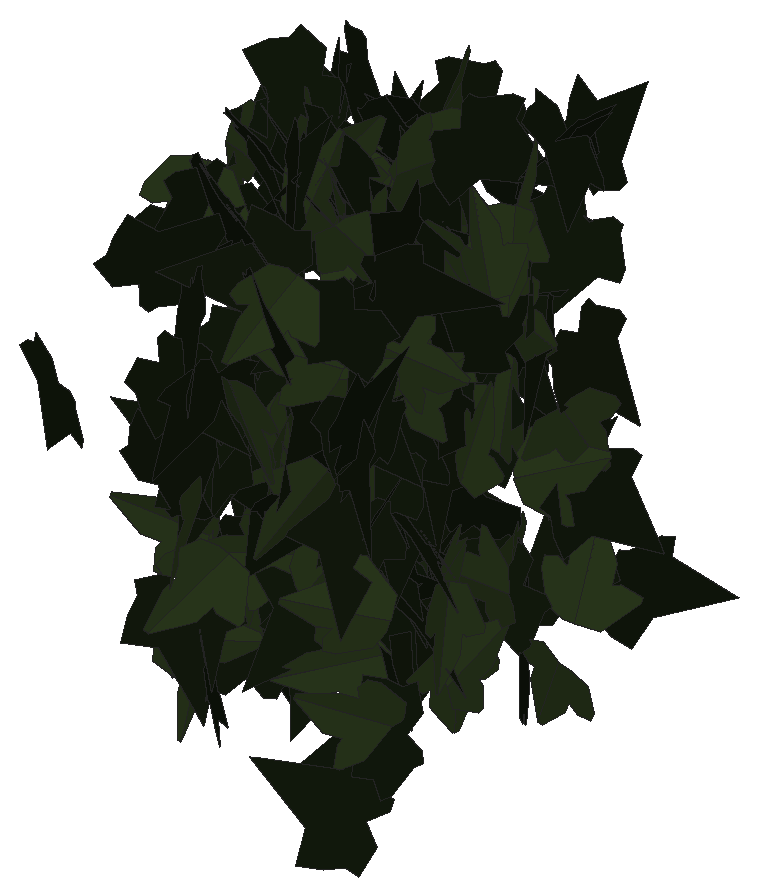
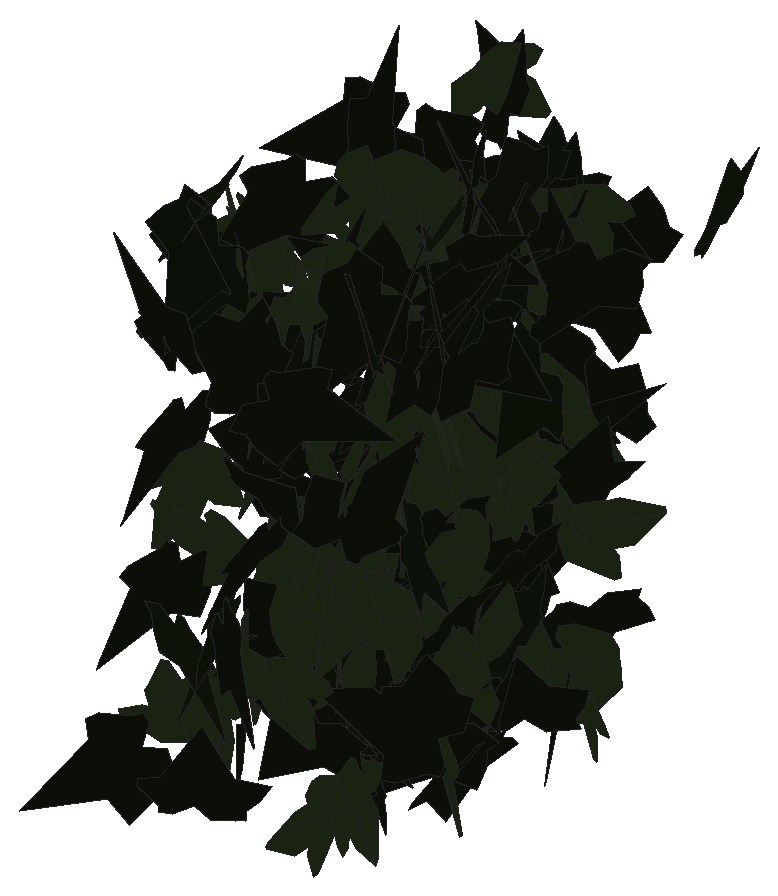
# SketchUp Ruby script. Lengths in inches.
U = 1.inch
M = Sketchup.active_model
def pt(a) = Geom::Point3d.new(a.map { |v| v * U })
def face(e, loops, mat)
  f = e.add_face(loops[0].map { |a| pt(a) })
  loops[1..].each { |l| e.add_face(l.map { |a| pt(a) }).erase! }
  f.material = f.back_material = mat if mat
  f
end
# faces: each face lists its corners as indices into pts; further lists are holes
def faces(e, pts, list, mat = nil) = list.each { |f| face(e, (f[0].is_a?(Array) ? f : [f]).map { |l| l.map { |i| pts[i] } }, mat) }
# xy, xz, yz: faces in a plane at the given z, y or x. An outline is a flat list of corners, or four numbers for a rectangle; further outlines are holes
def ring(l) = l.size == 4 ? [[l[0], l[1]], [l[2], l[1]], [l[2], l[3]], [l[0], l[3]]] : l.each_slice(2).to_a
def flat(e, list, mat, &to3) = list.each { |f| face(e, (f[0].is_a?(Array) ? f : [f]).map { |l| ring(l).map { |u, v| to3.(u, v) } }, mat) }
def xy(e, z, list, mat = nil) = flat(e, list, mat) { |x, y| [x, y, z] }
def xz(e, y, list, mat = nil) = flat(e, list, mat) { |x, z| [x, y, z] }
def yz(e, x, list, mat = nil) = flat(e, list, mat) { |y, z| [x, y, z] }
def lines(e, pts, list) = list.each { |a, b| e.add_line(pt(pts[a]), pt(pts[b])) }
# prism: a flat outline (further loops are holes) pulled along v
def prism(e, loops, v, mat = nil)
  f = face(e, loops, mat); d = Geom::Vector3d.new(v.map { |x| x * U })
  f.pushpull(f.normal.samedirection?(d) ? d.length : -d.length)
end
def box(e, o, s, mat = nil) = prism(e, [[o, [o[0] + s[0], o[1], o[2]], [o[0] + s[0], o[1] + s[1], o[2]], [o[0], o[1] + s[1], o[2]]]], [0, 0, s[2]], mat)
def at(x, y, z, deg = 0) = Geom::Transformation.translation(pt([x, y, z])) * Geom::Transformation.rotation(ORIGIN, Z_AXIS, deg.degrees)
def axes(o, x, y, z) = Geom::Transformation.new([*x, 0, *y, 0, *z, 0, *pt(o).to_a, 1])
def part(name) = M.definitions.add(name)
# library, detail: a bought-in or finely detailed component or shape, given as its bounding box
def library(name, o, s) = part(name).tap { |d| box(d.entities, o, s) }
def detail(e, o, s) = box(e.add_group.entities, o, s)
def put(e, d, t, mat = nil) = e.add_instance(d, t).tap { |i| i.material = mat if mat }
def group(e, t, mat = nil) = e.add_group.tap { |g| g.transformation = t; g.material = mat if mat }.entities
root = M.entities
M.materials.add("efeu1").color = [18, 25, 13]
M.materials.add("efeu2").color = [43, 57, 29]
c1 = part("ivyleaf_9")
p = [[1.54,2.16,1.25],[1.36,2.04,1.19],[-0.21,0.99,0.68],[-0.71,1.11,0.82],[-0.85,0.86,0.67],[-0.8,0.17,0.21],
  [-0.9,-0.01,0.1],[-0.67,-0.16,-0.02],[-0.08,-0.08,-0.05],[-0.03,-0.6,-0.4],[0.65,-0.88,-0.66],[0.83,-0.6,-0.49],
  [1.29,-0.42,-0.43],[1.8125,-0.07,-0.26],[1.21,0.44,0.15]]
faces(c1.entities,p,[[0,1,2,3,4,5,6,7,8,9,10,11,12,13,14]],"efeu1")
c2 = part("ivyleaf_10")
p = [[0,0.5,-0.03],[-0.0625,2.02,-0.43],[-0.19,2.01,-0.46],[-0.54,1.05,-0.29],[-0.52,0.625,-0.18],[-0.83,0.76,-0.28],
  [-1.16,0.64,-0.33],[-1.15,0.33,-0.24],[-0.77,-0.39,0.02],[-0.3,-0.51,0.16],[0.04,-0.48,0.23],[-0.02,2.01,-0.4375],
  [-0.06,2.01,-0.43],[0.04,-0.49,0.23],[0.67,-0.49,0.14],[1.38,0.36,-0.2],[1.375,0.51,-0.24],[0.81,0.65,-0.19],
  [0.62,0.59,-0.15],[0.6,1.09,-0.28],[0.5,1.23,-0.31]]
faces(c2.entities,p,[[0,1,2,3,4,5,6,7,8,9,10],[11,12,0,13,14,15,16,17,18,19,20]],"efeu2")
put(root,c1,axes([31.6875,223.98,213.96],[-0.33747,-0.32736,0.17014],[-0.11694,-0.12378,-0.47011],[0.34991,-0.35709,0.00698]))
put(root,c1,axes([31.4375,221.77,213.03],[-0.01587,-0.27679,-0.41609],[0.04585,0.41374,-0.27698],[0.49764,-0.04695,0.01225]))
put(root,c2,axes([31.33,222.96,213.41],[0.06539,-0.12843,-0.47878],[0.30609,-0.3694,0.14089],[-0.38991,-0.31152,0.03031]))
put(root,c1,axes([31.81,221.8,210.03],[-0.3415,-0.32972,0.15703],[0.11823,0.1036,0.47465],[-0.34554,0.36132,0.00721]))
put(root,c2,axes([31.98,221.37,209.31],[-0.14783,-0.03082,-0.47665],[-0.46593,-0.10055,0.151],[-0.10516,0.48881,0.00101]))
put(root,c2,axes([31.57,224.38,211.75],[0.2481,-0.43409,-0.00389],[0.0025,-0.00306,0.49998],[-0.4341,-0.24811,0.00065]))
put(root,c2,axes([31.63,222.88,210.6],[-0.00162,0.11657,-0.48622],[-0.04741,-0.48407,-0.11589],[-0.49774,0.04573,0.01262]))
put(root,c1,axes([31.56,224.39,209.48],[-0.06194,-0.46788,0.16508],[-0.02755,-0.16286,-0.47193],[0.49538,-0.06756,-0.0056]))
put(root,c1,axes([31.375,224.01,212.62],[0.48534,0.05286,-0.10793],[0.10585,0.02454,0.48805],[0.0569,-0.49659,0.01263]))
put(root,c1,axes([31.6875,224.75,210.8],[-0.29345,0.16275,-0.37067],[0.3272,-0.17423,-0.33554],[-0.23838,-0.43949,-0.00425]))
put(root,c2,axes([31.4,224.05,208.94],[0.3357,-0.12424,-0.3491],[0.3321,-0.10805,0.35782],[-0.16435,-0.47211,0.00998]))
put(root,c1,axes([31.87,223.68,212.84],[-0.0005,0.11983,-0.48543],[-0.0203,-0.48503,-0.11972],[-0.49959,0.01959,0.00535]))
put(root,c1,axes([31.8125,222.31,211.74],[0.04684,0.37913,0.3226],[0.03612,0.32058,-0.382],[-0.49649,0.05909,0.00264]))
put(root,c1,axes([31.875,225.68,211.17],[0.10776,0.10707,0.47636],[-0.43164,-0.2071,0.1442],[0.22819,-0.44232,0.0478]))
put(root,c1,axes([31.89,224.11,213.38],[-0.02238,-0.40573,-0.29134],[-0.01936,-0.29071,0.40634],[-0.49912,0.02947,-0.0027]))
put(root,c1,axes([31.54,224.39,213.21],[-0.03654,0.22317,0.44594],[0.07138,-0.44019,0.22614],[0.49353,0.08019,0.00031]))
put(root,c2,axes([31.41,225.27,210.07],[-0.21676,0.08364,-0.44274],[0.41102,-0.16459,-0.23232],[-0.1846,-0.46467,0.0026]))
put(root,c1,axes([31.57,222.9,209.77],[0.16919,-0.41329,-0.22487],[-0.08353,0.20879,-0.44658],[0.46303,0.18868,0.0016]))
put(root,c1,axes([31.86,224.08,212.77],[0.00119,-0.49676,0.05684],[0.03122,0.0568,0.49578],[-0.49902,0.00237,0.03115]))
put(root,c2,axes([31.78,223.5625,210.01],[0.05454,-0.15211,0.47317],[-0.11922,0.45811,0.16101],[-0.48251,-0.13038,0.0137]))
put(root,c2,axes([31.79,221.69,213.65],[0.44104,0.2007,-0.1233],[-0.11246,-0.05056,-0.48456],[-0.20697,0.45515,0.00054]))
put(root,c2,axes([31.75,222.37,210.68],[0.03924,0.41759,0.27217],[0.01727,0.27171,-0.41937],[-0.49816,0.04231,0.0069]))
put(root,c2,axes([31.79,221.63,207.48],[0.4189,-0.26458,0.06722],[0.05738,-0.03504,-0.49546],[0.26689,0.42281,0.00101]))
put(root,c1,axes([31.6,220.93,212.64],[-0.04412,-0.02615,0.49736],[0.48102,0.1272,0.04936],[-0.12911,0.48284,0.01393]))
put(root,c1,axes([31.58,223,208.71],[0.06296,-0.27116,0.41534],[0.15597,-0.38662,-0.27605],[0.47086,0.16432,0.0359]))
put(root,c1,axes([31.99,221.86,213.51],[-0.02515,0.05008,-0.49685],[0.05384,-0.49431,-0.05255],[-0.49646,-0.05614,0.01947]))
put(root,c2,axes([32.01,223.83,207.62],[0.30138,-0.30171,-0.26104],[-0.17078,0.19809,-0.42614],[0.36056,0.34602,0.01635]))
put(root,c1,axes([31.86,224.37,214.11],[0.30513,-0.19859,-0.34272],[-0.29281,0.17825,-0.36399],[0.26675,0.42283,-0.00752]))
put(root,c2,axes([31.85,225.26,211.94],[-0.14818,0.46373,-0.11399],[0.03283,-0.10917,-0.48683],[-0.47641,-0.15176,0.0019]))
put(root,c1,axes([31.58,223.63,213.24],[0.27836,-0.32305,0.26106],[0.18025,-0.18917,-0.42629],[0.37419,0.33144,0.01115]))
put(root,c1,axes([31.53,224.53,208.22],[0.21128,-0.08624,0.44489],[0.44522,-0.05202,-0.22152],[0.08449,0.48975,0.05481]))
put(root,c2,axes([31.98,224.79,212.15],[-0.03583,-0.15054,-0.47545],[-0.12988,-0.45741,0.15462],[-0.48151,0.13458,-0.00633]))
put(root,c2,axes([32,225.25,212.0625],[-0.2445,0.39048,0.19429],[-0.10854,0.16125,-0.46067],[-0.42242,-0.26744,0.00592]))
put(root,c1,axes([31.8125,221.43,208.35],[-0.10098,-0.44105,-0.21278],[0.05253,0.20625,-0.45244],[0.48687,-0.11373,0.00468]))
put(root,c1,axes([31.79,223.7,207.39],[0.03275,-0.49311,-0.07595],[-0.00644,0.07569,-0.4942],[0.49888,0.03335,-0.00139]))
put(root,c2,axes([31.93,225.46,210.32],[-0.1341,-0.40709,-0.25748],[0.10901,0.23469,-0.42783],[0.46918,-0.17088,0.02581]))
put(root,c2,axes([31.65,221.5,207.76],[-0.04159,-0.0317,-0.49726],[0.44458,0.22294,-0.0514],[0.22498,-0.44642,0.00965]))
put(root,c2,axes([32.05,226.7,209.76],[0.46811,0.08876,-0.15165],[-0.14956,-0.02529,-0.47644],[-0.09225,0.49141,0.00288]))
put(root,c2,axes([31.8125,221.9,210.1],[0.36867,-0.20175,0.27089],[0.23709,-0.13104,-0.42026],[0.24057,0.43832,-0.00096]))
put(root,c2,axes([31.63,221.86,211.14],[0.16871,0.04916,0.4681],[0.45456,0.11199,-0.17559],[-0.12211,0.48481,-0.0069]))
put(root,c1,axes([31.875,224.4,212.93],[0.49003,0.0694,-0.07107],[-0.07051,-0.00894,-0.49492],[-0.06996,0.49508,0.00102]))
put(root,c2,axes([31.96,223.61,213.27],[-0.20873,0.26397,0.36979],[0.21214,-0.30325,0.33621],[0.40178,0.29725,0.0146]))
put(root,c1,axes([32.36,221.36,210.33],[-0.22809,-0.41409,-0.16281],[-0.08117,-0.14116,0.47274],[-0.43748,0.24208,-0.00283]))
put(root,c1,axes([31.87,219.02,212.21],[0.02308,-0.31051,0.39122],[0.0806,-0.38419,-0.30968],[0.49292,0.07735,0.03232]))
put(root,c1,axes([32.1875,221.34,207.61],[0.24178,-0.08541,-0.42924],[-0.4062,0.13877,-0.25641],[0.16293,0.4727,-0.00228]))
put(root,c1,axes([31.96,223.8,210.49],[0.09241,-0.38341,-0.30734],[-0.05194,0.30335,-0.39406],[0.48863,0.10476,0.01624]))
put(root,c1,axes([32.37,226.28,212.93],[-0.03093,-0.07972,-0.49263],[-0.15258,-0.46843,0.08538],[-0.47515,0.15561,0.00465]))
put(root,c1,axes([32.16,222.12,207.2],[-0.4058,-0.04412,0.28876],[0.28662,0.03526,0.40818],[-0.05638,0.4968,-0.00333]))
put(root,c1,axes([31.93,223.86,207.87],[-0.04751,-0.19126,-0.45952],[0.19265,0.41857,-0.19413],[0.45894,-0.1955,0.03392]))
put(root,c2,axes([32.19,225.22,207.53],[0.09483,-0.45348,0.18806],[0.05034,-0.18155,-0.46315],[0.48834,0.10677,0.01122]))
put(root,c2,axes([31.87,222.99,208.96],[0.11348,0.03298,0.48583],[0.36113,0.32894,-0.10669],[-0.32666,0.37511,0.05084]))
put(root,c2,axes([32.43,225.9,209.875],[-0.4175,0.14422,-0.2343],[-0.2266,0.06126,0.44147],[0.15605,0.47481,0.0142]))
put(root,c2,axes([32.19,222.73,211.33],[-0.24883,-0.3895,-0.19071],[0.10731,0.15774,-0.46217],[0.4202,-0.27094,0.00509]))
put(root,c1,axes([32.35,221.53,211.53],[-0.154,0.38706,-0.27652],[0.10227,-0.25692,-0.41657],[-0.46457,-0.18486,-0.00004]))
put(root,c1,axes([32.47,224.46,213.02],[-0.03666,0.2016,0.45609],[-0.11952,0.44043,-0.20429],[-0.48412,-0.124,0.0159]))
put(root,c2,axes([32.58,224.46,209.41],[0.06373,0.0427,0.49408],[-0.41244,-0.27205,0.07671],[0.27538,-0.41733,0.00055]))
put(root,c1,axes([32.07,222.75,209.68],[-0.01929,-0.25091,-0.43206],[0.055,0.42868,-0.25141],[0.49659,-0.05722,0.01106]))
put(root,c1,axes([31.9,222.42,213.97],[0.41904,-0.21858,0.16318],[0.14463,-0.07556,-0.47262],[0.23127,0.4433,-0.0001]))
put(root,c2,axes([32.1,223.68,213.03],[-0.2701,-0.3327,0.25759],[0.19936,0.16837,0.42651],[-0.37054,0.33311,0.0417]))
put(root,c1,axes([32.32,221.41,210.54],[-0.43596,-0.1124,-0.21751],[0.21411,0.04043,-0.45003],[0.11875,-0.48552,0.01288]))
put(root,c1,axes([32.13,221.8,212.71],[0.11235,0.47958,0.08593],[-0.02714,-0.08189,0.4925],[0.48646,-0.11533,0.00763]))
put(root,c1,axes([32,221.66,213.42],[0.10812,-0.15471,0.46301],[0.24512,-0.39291,-0.18852],[0.42217,0.26775,-0.00912]))
put(root,c1,axes([32.07,220.67,210.29],[-0.11941,0.02304,0.48499],[0.38859,-0.29491,0.10968],[0.29111,0.40311,0.05253]))
put(root,c1,axes([32.23,223.34,212.66],[0.14247,-0.39845,-0.26634],[-0.09261,0.24974,-0.42315],[0.47024,0.1699,-0.00264]))
put(root,c2,axes([32.46,223.6,212.4375],[-0.23014,-0.44384,0.00672],[-0.00044,-0.00734,-0.49995],[0.44389,-0.23012,0.00298]))
put(root,c2,axes([32.6875,222.01,208.51],[-0.02885,0.05399,-0.49624],[-0.32861,0.37211,0.05959],[0.37574,0.32958,0.01401]))
put(root,c2,axes([32.17,224.34,210.4],[0.01671,-0.09724,-0.49017],[0.22804,-0.43492,0.09405],[-0.44466,-0.2267,0.02981]))
put(root,c2,axes([32.46,223.84,210.76],[-0.46503,-0.18333,-0.01159],[0.01082,0.00415,-0.49987],[0.18337,-0.46516,0.00011]))
put(root,c2,axes([32.66,225.24,211.84],[0.1745,-0.14908,-0.44421],[-0.32763,0.30005,-0.2294],[0.33497,0.37114,0.00704]))
put(root,c1,axes([32.29,224.57,213.51],[0.47579,0.13317,-0.07676],[-0.07397,-0.02051,-0.49407],[-0.13474,0.4815,0.00019]))
put(root,c1,axes([32.02,223.64,212.79],[0.27165,-0.04267,0.4176],[0.4118,-0.06937,-0.27497],[0.08141,0.49332,-0.00255]))
put(root,c2,axes([32.27,221.85,212.14],[0.01431,-0.14824,0.4773],[0.29289,-0.38443,-0.12818],[0.40498,0.28327,0.07583]))
put(root,c1,axes([32.74,226.7,210.07],[0.04767,0.02892,-0.49688],[-0.49746,0.01905,-0.04662],[0.01623,0.4988,0.03059]))
put(root,c1,axes([32.37,224.19,208.59],[0.02113,0.17867,0.46651],[-0.10826,-0.45419,0.17885],[0.48768,-0.10857,0.0195]))
put(root,c1,axes([32.32,223.51,209.57],[0.07971,-0.45237,-0.19751],[-0.01439,0.19785,-0.45896],[0.4934,0.07885,0.01852]))
put(root,c2,axes([32.39,222.86,210.62],[-0.14962,-0.22597,-0.42018],[0.22559,0.35451,-0.27098],[0.42039,-0.27066,-0.00413]))
put(root,c2,axes([32.41,222.16,208.12],[-0.35618,-0.24888,-0.24738],[0.20595,0.13712,-0.43449],[0.28411,-0.41141,0.00483]))
put(root,c1,axes([32.71,223.81,208.06],[-0.4195,-0.2182,0.16251],[-0.13959,-0.08375,-0.47276],[0.23353,-0.44201,0.00935]))
put(root,c1,axes([32.21,222.49,213.57],[0.17939,-0.34883,0.31006],[0.1287,-0.28232,-0.39209],[0.44862,0.22048,-0.0115]))
put(root,c2,axes([32.4,223.46,212.85],[-0.32131,0.20455,0.32391],[0.24847,-0.2105,0.37941],[0.29159,0.40478,0.03362]))
put(root,c2,axes([32.26,222.0625,208.2],[-0.28007,-0.0433,-0.41193],[0.41419,-0.02526,-0.27895],[0.00335,-0.49748,0.05002]))
put(root,c2,axes([32.36,223.17,211.46],[0.19044,-0.26004,0.38225],[0.26819,-0.2746,-0.32042],[0.37657,0.32707,0.03489]))
put(root,c1,axes([32.19,220.55,211.88],[0.03481,-0.09503,-0.48965],[0.40967,0.28544,-0.02628],[0.28453,-0.39936,0.09774]))
put(root,c2,axes([32.49,222.44,212.73],[0.11833,-0.44434,0.19637],[-0.00038,0.20202,0.45737],[-0.4858,-0.10839,0.04747]))
put(root,c1,axes([32.78,222.28,207.125],[0.12558,-0.16279,0.45577],[-0.24015,0.38785,0.2047],[-0.42019,-0.27032,0.01923]))
put(root,c2,axes([32.37,222.22,209.77],[-0.16775,0.12511,0.4541],[0.36679,-0.26773,0.20926],[0.29551,0.40332,-0.00195]))
put(root,c1,axes([32.45,222.33,213.28],[-0.18475,0.32714,0.32992],[0.16552,-0.28541,0.37569],[0.43413,0.24803,-0.00284]))
put(root,c1,axes([32.3,221.93,209.14],[-0.06821,-0.0309,-0.49436],[0.46072,0.17929,-0.07477],[0.18188,-0.46573,0.00401]))
put(root,c2,axes([32.82,223.28,212.34],[0.20634,-0.12625,-0.43759],[-0.22357,0.39046,-0.21808],[0.39679,0.28566,0.10468]))
put(root,c1,axes([32.37,223.51,213.66],[0.19987,-0.44368,0.11491],[0.06452,-0.09687,-0.48626],[0.45375,0.2092,0.01853]))
put(root,c2,axes([32.28,224.28,213.01],[0.19035,0.0062,-0.46231],[0.45848,0.06203,0.18961],[0.0597,-0.4961,0.01793]))
put(root,c1,axes([32.52,223.61,209.82],[-0.09522,-0.04269,0.48899],[0.03825,-0.49724,-0.03596],[0.48936,0.03056,0.09796]))
put(root,c1,axes([32.27,223.51,209.3],[0.10871,-0.13891,0.46785],[0.35515,-0.30623,-0.17345],[0.33473,0.37003,0.03209]))
put(root,c2,axes([32.97,221.59,209.24],[-0.00853,-0.0025,-0.49992],[-0.45122,-0.21524,0.00877],[-0.21525,0.45129,0.00142]))
put(root,c1,axes([32.31,221.6,213.6],[0.27934,-0.33083,0.25004],[0.16397,-0.18879,-0.43298],[0.3809,0.3239,0.00302]))
put(root,c2,axes([32.64,223.625,210.55],[0.14155,-0.42719,0.21789],[0.07218,-0.20562,-0.45001],[0.47408,0.15885,0.00346]))
put(root,c2,axes([32.76,223.6,209.59],[-0.08134,-0.42567,0.24938],[-0.04213,-0.24584,-0.43335],[0.49154,-0.09151,0.00413]))
put(root,c2,axes([32.78,222.11,209.9],[-0.07693,-0.39941,0.29078],[-0.06321,-0.28391,-0.40669],[0.48999,-0.09934,-0.00681]))
put(root,c2,axes([32.34,222.86,207.47],[-0.1561,-0.06611,0.47038],[0.42912,0.1927,0.16949],[-0.2037,0.45661,-0.00342]))
put(root,c2,axes([32.75,225.05,212.8],[0.14936,-0.33311,-0.34165],[-0.05252,0.34435,-0.3587],[0.47427,0.14304,0.06788]))
put(root,c1,axes([32.91,225.21,211.64],[-0.15928,-0.44468,-0.164],[-0.02968,-0.16331,0.47164],[-0.47302,0.15998,0.02563]))
put(root,c1,axes([32.74,222.875,211.1],[-0.4304,-0.19261,-0.16631],[0.14981,0.07237,-0.47151],[0.20571,-0.4557,-0.00459]))
put(root,c1,axes([32.5625,223.65,210.91],[0.25789,-0.30356,-0.30223],[-0.14343,0.27121,-0.3948],[0.40363,0.29033,0.05281]))
put(root,c2,axes([32.73,222.45,213.28],[0.03913,0.29118,-0.40458],[0.05873,0.40031,0.29378],[0.495,-0.07051,-0.00287]))
put(root,c1,axes([32.8125,222.92,207.92],[-0.46924,0.08955,0.14762],[0.14173,-0.04436,0.47743],[0.09861,0.48991,0.01625]))
put(root,c1,axes([32.56,220.62,212.96],[-0.20497,0.00829,-0.45598],[0.44937,-0.08157,-0.20349],[-0.07777,-0.49323,0.02599]))
put(root,c2,axes([32.59,225.47,213.49],[0.0345,-0.10263,-0.48814],[0.12146,-0.47285,0.108],[-0.4838,-0.12603,-0.00769]))
put(root,c1,axes([32.56,222.54,213.96],[-0.03112,0.0256,-0.49837],[0.44092,-0.23245,-0.03947],[-0.23372,-0.44194,-0.00811]))
put(root,c2,axes([33.02,223.31,212.61],[0.22774,-0.10108,0.43349],[-0.40091,0.165,0.24909],[-0.19341,-0.46104,-0.00589]))
put(root,c2,axes([32.75,224.92,207.01],[0.01089,-0.01603,-0.49962],[0.10552,0.48855,-0.01338],[0.48862,-0.10515,0.01402]))
put(root,c2,axes([32.79,224.21,208.4],[-0.05152,0.21142,0.45016],[0.07227,-0.44459,0.21707],[0.49206,0.08743,0.01526]))
put(root,c1,axes([32.54,221.29,209.36],[0.00747,0.07415,-0.49441],[0.15253,0.47056,0.07288],[0.47611,-0.15191,-0.01559]))
put(root,c2,axes([32.64,220.54,210.19],[0.16249,-0.23272,0.41163],[0.23418,-0.33853,-0.28383],[0.4108,0.28503,-0.00102]))
put(root,c2,axes([32.875,222.26,207.77],[-0.06235,0.47883,-0.12973],[-0.03758,0.12582,0.48245],[0.49467,0.06991,0.0203]))
put(root,c2,axes([32.56,222.66,211.5625],[-0.12265,0.00553,0.48469],[0.37173,-0.31979,0.09771],[0.31108,0.38432,0.07433]))
put(root,c1,axes([32.69,221.66,213.08],[-0.3346,-0.16843,-0.33117],[0.30099,0.13841,-0.3745],[0.21783,-0.44997,0.00877]))
put(root,c2,axes([32.8,224.36,210.07],[-0.10011,-0.10075,0.4794],[0.11255,-0.48095,-0.07757],[0.47677,0.09239,0.11897]))
put(root,c2,axes([33.17,221.43,210.71],[0.09338,-0.02897,0.49035],[-0.48159,0.09286,0.0972],[-0.0967,-0.49045,-0.01056]))
put(root,c1,axes([32.63,224.46,211.33],[0.11457,-0.46802,0.13353],[0.03053,-0.12999,-0.48184],[0.48574,0.11856,-0.00121]))
put(root,c2,axes([32.6,223.68,209.96],[-0.318,0.04135,0.38362],[0.37859,-0.06252,0.32057],[0.07448,0.49435,0.00845]))
put(root,c1,axes([32.49,224.23,213.23],[0.15508,-0.09379,0.466],[0.40961,-0.22235,-0.18107],[0.24119,0.43791,0.00787]))
put(root,c1,axes([32.88,221.34,212.08],[-0.26922,-0.4162,-0.06554],[0.03627,0.0546,-0.49569],[0.41977,-0.27165,0.00079]))
put(root,c1,axes([33.03,221.95,212.46],[-0.37416,-0.31537,0.10271],[-0.07155,-0.07444,-0.48922],[0.32386,-0.38079,0.01057]))
put(root,c2,axes([32.98,222.71,211.4],[0.11426,-0.22119,0.43361],[-0.1747,0.39709,0.24859],[-0.45434,-0.20831,0.01346]))
put(root,c1,axes([33.3125,221.33,213.08],[-0.29966,-0.02149,0.39967],[-0.39787,-0.03839,-0.30038],[0.0436,-0.49806,0.00591]))
put(root,c1,axes([32.85,222.78,207.78],[-0.14687,-0.09115,0.46917],[0.38019,0.27516,0.17247],[-0.28963,0.40741,-0.01152]))
put(root,c1,axes([32.69,225.14,208.22],[-0.13775,-0.20239,-0.43596],[0.34226,0.27711,-0.23678],[0.33747,-0.36366,0.0622]))
put(root,c1,axes([33.06,220.41,212.1],[-0.05738,0.29272,-0.40127],[0.09422,-0.39019,-0.29811],[-0.48768,-0.10983,-0.01038]))
put(root,c1,axes([33.26,225.42,211.01],[-0.47459,0.03056,-0.15436],[-0.1544,0.00427,0.47555],[0.03038,0.49905,0.00538]))
put(root,c2,axes([33.11,220.29,209.66],[0.27006,0.22931,-0.35282],[-0.28211,-0.21239,-0.35398],[-0.31222,0.39026,0.01466]))
put(root,c2,axes([33.29,221.47,210.4],[-0.22213,0.1689,-0.41489],[-0.32892,0.25288,0.27905],[0.30409,0.3969,-0.00123]))
put(root,c1,axes([32.76,224.14,207.37],[-0.15994,-0.02885,-0.47285],[0.47349,-0.02572,-0.15859],[-0.01517,-0.4985,0.03555]))
put(root,c2,axes([32.96,223.3,211.58],[0.07367,-0.15725,-0.46888],[0.09708,0.46943,-0.14218],[0.48492,-0.07009,0.09969]))
put(root,c1,axes([32.84,222.21,208.75],[0.09422,-0.35059,-0.34382],[-0.00505,0.34938,-0.35764],[0.49102,0.07087,0.0623]))
put(root,c1,axes([32.97,224.12,207.62],[-0.36904,-0.13074,-0.311],[0.29784,0.09023,-0.39135],[0.15845,-0.4741,0.01128]))
put(root,c1,axes([32.85,222.8,210.64],[-0.21314,0.0726,0.44643],[0.39779,-0.20479,0.22322],[0.21526,0.45032,0.02954]))
put(root,c2,axes([33.09,223.46,209.55],[-0.35228,0.35413,0.02224],[-0.01736,0.01409,-0.4995],[-0.3544,-0.3527,0.00237]))
put(root,c2,axes([32.95,221.7,212.24],[-0.21009,0.36617,-0.26792],[0.13783,-0.2298,-0.42213],[-0.43228,-0.25122,-0.00438]))
put(root,c1,axes([33.05,223.88,206.79],[-0.01755,0.11311,0.48672],[-0.1472,-0.46658,0.10313],[0.47752,-0.13967,0.04968]))
put(root,c1,axes([33.1,223.71,207.625],[-0.16756,0.47056,0.0222],[0.00707,-0.02105,0.49951],[0.47103,0.16771,0.0004]))
put(root,c2,axes([33.48,221.56,212.51],[-0.27315,0.15775,-0.38795],[-0.33494,0.19575,0.31543],[0.25139,0.4322,-0.00126]))
put(root,c2,axes([33.01,224.19,213.39],[-0.1372,-0.16329,-0.45223],[0.30718,0.33202,-0.21308],[0.36989,-0.3363,0.00921]))
put(root,c1,axes([33.24,222.19,209.38],[-0.43922,-0.16211,-0.17551],[0.16276,0.06587,-0.46816],[0.17491,-0.46838,-0.00509]))
put(root,c1,axes([33.5,222.34,212.35],[-0.45402,0.20405,0.04724],[-0.04393,0.01748,-0.49776],[-0.20478,-0.45613,0.00205]))
put(root,c1,axes([33.01,222.62,209.68],[-0.15855,-0.06959,0.46906],[0.32907,-0.37226,0.056],[0.34143,0.32647,0.16384]))
put(root,c2,axes([33.125,221.58,210.79],[0.23514,-0.2941,0.32896],[0.19624,-0.26417,-0.37644],[0.39522,0.30614,-0.00881]))
put(root,c1,axes([32.96,223.67,208.4],[0.42709,0.06859,0.25079],[0.24827,0.0356,-0.43254],[-0.07719,0.49399,-0.00365]))
put(root,c1,axes([33.01,222.75,211.03],[0.47541,0.05068,0.14634],[0.1441,0.02835,-0.47794],[-0.05674,0.49662,0.01235]))
put(root,c1,axes([33.17,225.4375,210.6],[0.22187,-0.32604,-0.30736],[-0.13747,0.27691,-0.39297],[0.42647,0.25888,0.03323]))
put(root,c2,axes([32.95,222.75,209.61],[0.02275,-0.06038,0.49582],[0.4977,0.04469,-0.0174],[-0.04221,0.49432,0.06214]))
put(root,c2,axes([33.7,224.39,209.97],[0.0646,-0.0275,-0.49505],[-0.4611,0.18016,-0.07018],[0.18224,0.4656,-0.00209]))
put(root,c2,axes([33.29,224.48,209.85],[-0.27553,0.39603,-0.13131],[0.07484,-0.1079,-0.48245],[-0.41047,-0.28551,0.00018]))
put(root,c2,axes([33.4375,223.69,208.65],[0.14155,-0.38047,-0.2919],[-0.04259,0.29317,-0.40279],[0.47765,0.13889,0.05059]))
put(root,c1,axes([33.625,222.79,212.58],[-0.41556,0.27552,-0.03735],[0.03021,-0.02203,-0.4986],[-0.2764,-0.41666,0.00166]))
put(root,c1,axes([33.49,221.93,208.68],[-0.30914,-0.34877,0.18109],[-0.11323,-0.14158,-0.46598],[0.37631,-0.32911,0.00855]))
put(root,c1,axes([33.625,221.25,210.35],[0.13237,0.26591,-0.40221],[-0.18202,-0.35866,-0.29703],[-0.44648,0.22506,0.00185]))
put(root,c2,axes([33.13,222.61,210.2],[0.32099,-0.03879,0.38139],[0.37515,-0.0706,-0.32292],[0.07891,0.49347,-0.01622]))
put(root,c1,axes([33.43,222.15,208.27],[-0.22,-0.44688,0.04362],[-0.01896,-0.03929,-0.49809],[0.4486,-0.22081,0.00034]))
put(root,c2,axes([33.4,221.76,209],[0.05117,0.19387,-0.45804],[0.13841,0.43671,0.20031],[0.47773,-0.14729,-0.00897]))
put(root,c1,axes([33.36,222.84,209.1],[0.35227,-0.30553,-0.18043],[-0.13578,0.11882,-0.46631],[0.32782,0.37753,0.00074]))
put(root,c2,axes([33.58,222.91,210.46],[0.116,-0.13825,-0.46629],[0.00095,0.47944,-0.14191],[0.48636,0.03204,0.11149]))
put(root,c1,axes([33.59,224.42,208.65],[0.39215,-0.11472,0.2882],[-0.27728,0.07859,0.40858],[-0.13904,-0.48027,-0.00198]))
put(root,c2,axes([33.36,222.6875,211.17],[0.14213,-0.21633,0.42779],[0.29441,-0.31273,-0.25597],[0.37831,0.32465,0.03848]))
put(root,c1,axes([33.35,222.87,208.7],[-0.19471,-0.17249,-0.42701],[0.33161,0.26919,-0.25995],[0.31957,-0.38443,0.00957]))
put(root,c2,axes([33.3,222.64,212.96],[0.36458,0.16969,0.29713],[0.27095,0.12197,-0.40213],[-0.20896,0.45423,-0.00302]))
put(root,c1,axes([33.6,223.61,208.77],[0.32734,-0.35818,0.12066],[-0.07974,0.09058,0.48522],[-0.36945,-0.3369,0.00218]))
put(root,c2,axes([33.5,222.4375,211.77],[-0.4443,0.04003,0.22582],[0.21347,-0.1078,0.4391],[0.08384,0.4866,0.0787]))
put(root,c1,axes([33.59,224.16,212.37],[0.4129,0.00105,-0.28198],[-0.28095,0.04432,-0.41122],[0.02413,0.49803,0.03719]))
put(root,c2,axes([33.4375,222.78,208.17],[0.18192,0.29636,0.35927],[0.18386,0.30868,-0.34773],[-0.4279,0.25863,0.00333]))
put(root,c1,axes([33.59,225.56,209.58],[0.36894,-0.16985,-0.29161],[-0.2609,0.13049,-0.40608],[0.21405,0.4518,0.00766]))
put(root,c1,axes([33.8,223.6,212.69],[-0.07167,-0.41879,0.26359],[0.04675,0.25941,0.42487],[-0.49262,0.08555,0.00197]))
put(root,c1,axes([33.59,220.97,210.6],[0.22515,0.33863,0.29092],[0.15626,0.24544,-0.40662],[-0.4182,0.27402,0.0047]))
put(root,c1,axes([33.27,223.91,212.31],[0.19274,-0.09151,0.45219],[0.44968,-0.07232,-0.2063],[0.10316,0.48621,0.05442]))
put(root,c2,axes([33.77,223.93,212.14],[-0.24012,-0.35909,-0.25179],[-0.14229,-0.20775,0.43196],[-0.41485,0.2791,-0.00242]))
put(root,c2,axes([33.62,220.18,212.11],[-0.41701,0.21791,-0.16918],[0.14729,-0.08341,-0.47048],[-0.23326,-0.44222,0.00537]))
put(root,c1,axes([33.5,222.73,208.52],[0.46765,0.15714,0.08132],[-0.07687,-0.02654,0.49334],[0.15936,-0.47392,-0.00066]))
put(root,c1,axes([33.71,222.85,210.67],[-0.17026,0.15953,-0.44222],[0.28788,-0.33646,-0.23221],[-0.37167,-0.33368,0.02272]))
put(root,c2,axes([33.68,223.125,213.87],[-0.02684,-0.11616,-0.48558],[0.11438,0.47192,-0.11921],[0.486,-0.11748,0.00124]))
put(root,c1,axes([33.84,225.84,207.14],[-0.44038,-0.14127,0.19001],[0.18884,0.03251,0.46183],[-0.14284,0.47852,0.02472]))
put(root,c2,axes([34.1,221.72,208.2],[0.11296,0.06721,-0.48241],[-0.43389,-0.21114,-0.13102],[-0.22132,0.44822,0.01062]))
put(root,c2,axes([33.5,223.26,212.55],[0.26991,-0.10459,0.40769],[0.39622,-0.10024,-0.28803],[0.14198,0.47855,0.02877]))
put(root,c1,axes([33.58,222.81,209.26],[0.2526,-0.43114,0.01771],[0.00886,-0.01534,-0.49969],[0.43141,0.25275,-0.00011]))
put(root,c2,axes([33.68,222.11,213.41],[-0.37642,-0.13,-0.30233],[0.28291,0.10684,-0.39818],[0.16813,-0.47084,-0.00687]))
put(root,c2,axes([33.97,223.375,207.62],[0.25184,-0.26279,0.34281],[-0.23947,0.24531,0.36397],[-0.35948,-0.34751,-0.0023]))
put(root,c1,axes([33.72,221.42,211.57],[0.00002,-0.00406,-0.49998],[0.371,-0.33519,0.00274],[-0.3352,-0.37099,0.003]))
put(root,c1,axes([34.29,224.08,210.22],[-0.31548,-0.157,-0.35472],[-0.3032,-0.18538,0.35171],[-0.24195,0.43702,0.02176]))
put(root,c1,axes([33.78,222.43,210.93],[0.10175,-0.18594,-0.45285],[-0.12581,0.43706,-0.20773],[0.47309,0.15622,0.04216]))
put(root,c1,axes([33.5,225.24,212.375],[0.11636,-0.11912,0.47145],[0.38938,-0.26755,-0.16371],[0.29128,0.40525,0.0305]))
put(root,c1,axes([33.8,223.39,210.11],[-0.31738,-0.0604,-0.38161],[0.37152,0.08783,-0.32289],[0.10603,-0.48851,-0.01087]))
put(root,c1,axes([34.26,225.66,209.1],[-0.2804,0.40187,0.09937],[-0.05742,0.08111,-0.49003],[-0.40997,-0.28622,0.00066]))
put(root,c1,axes([33.81,222.86,209.77],[0.03385,-0.47357,0.15679],[0.01955,-0.15577,-0.47471],[0.49847,0.03827,0.00797]))
put(root,c2,axes([34.05,220.9,210.82],[-0.03377,-0.32857,0.37537],[-0.00453,-0.37601,-0.32954],[0.49884,-0.02566,0.02242]))
put(root,c1,axes([33.78,224.26,210.98],[0.46865,0.15266,0.08404],[-0.07979,-0.0264,0.49289],[0.15492,-0.47539,-0.00038]))
put(root,c1,axes([33.89,223.59,211.78],[0.06313,-0.13785,-0.47646],[0.33426,-0.34303,0.14353],[-0.36645,-0.33665,0.04885]))
put(root,c2,axes([34.15,220.99,212.41],[-0.03453,0.28376,0.41023],[-0.07134,-0.40979,0.27745],[0.49368,-0.03937,0.06879]))
put(root,c1,axes([33.9,223.9,214.09],[0.04618,-0.09673,-0.48837],[-0.00512,0.49035,-0.09761],[0.49784,0.01402,0.0443]))
put(root,c1,axes([34.15,223.03,207.42],[-0.16683,-0.24368,0.40347],[0.23661,0.32687,0.29525],[-0.40766,0.28944,0.00625]))
put(root,c1,axes([34.21,221.72,209.8125],[0.03816,0.28411,0.40966],[0.05657,0.40574,-0.28666],[-0.49532,0.06823,-0.00118]))
put(root,c1,axes([34.2,222.09,210.71],[-0.37746,-0.32734,0.01929],[-0.01416,-0.01312,-0.49963],[0.3276,-0.37773,0.00064]))
put(root,c2,axes([34.17,224.375,208.55],[0.09081,-0.47017,-0.14386],[-0.00334,0.1457,-0.47829],[0.49167,0.08783,0.02332]))
put(root,c1,axes([34.32,224.33,208.1],[-0.33892,-0.25771,0.26214],[-0.19445,-0.1769,-0.42532],[0.31196,-0.39024,0.01969]))
put(root,c2,axes([33.89,221.73,211.83],[-0.08584,-0.04311,-0.49069],[0.39502,0.29152,-0.09472],[0.29426,-0.40393,-0.01599]))
put(root,c2,axes([34.26,220.15,213.73],[0.24625,0.27554,-0.3368],[-0.22348,-0.25198,-0.36954],[-0.37339,0.33254,-0.00095]))
put(root,c2,axes([33.96,222.3,212.7],[0.04212,-0.04373,0.4963],[0.32159,-0.37803,-0.0606],[0.38054,0.32431,-0.00372]))
put(root,c2,axes([33.98,223.4375,208.43],[0.24676,-0.32128,-0.29306],[0.18859,-0.22456,0.40498],[-0.39184,-0.3104,0.01035]))
put(root,c1,axes([34.02,226.01,212.89],[-0.16676,0.21316,0.42042],[0.27425,-0.31883,0.27043],[0.38338,0.3208,-0.01058]))
put(root,c1,axes([34.13,221.52,211.68],[0.17811,-0.2672,-0.38325],[-0.13821,0.36167,-0.31638],[0.44629,0.21864,0.05497]))
put(root,c2,axes([34.19,221.72,210.75],[-0.13078,0.46139,-0.14147],[0.03352,-0.13753,-0.47954],[-0.48143,-0.13491,0.00504]))
put(root,c1,axes([34.53,221.02,213.21],[0.03743,0.05983,-0.49499],[-0.23832,-0.43387,-0.07046],[-0.43795,0.24121,-0.00397]))
put(root,c1,axes([33.97,223.6,211.47],[0.03635,0.01331,0.4985],[0.48903,0.0969,-0.03824],[-0.09763,0.49034,-0.00598]))
put(root,c1,axes([34.4,224.35,206.65],[0.04247,-0.17056,0.46809],[0.00503,0.46991,0.17076],[-0.49817,-0.0098,0.04163]))
put(root,c2,axes([34.31,224.03,212.45],[0.04119,-0.05949,0.49474],[-0.11605,0.48163,0.06757],[-0.4846,-0.1204,0.02587]))
put(root,c1,axes([33.97,222.74,209.59],[0.25872,-0.35556,0.23799],[0.14792,-0.18664,-0.43964],[0.40148,0.2979,0.00861]))
put(root,c2,axes([34.6875,223.53,208.56],[-0.07894,0.01116,0.4936],[-0.4936,0.00976,-0.07916],[-0.0114,-0.49978,0.00948]))
put(root,c2,axes([34.42,223.87,210.36],[0.01599,0.33618,-0.36976],[-0.05573,0.36885,0.33294],[0.49663,0.03056,0.04927]))
put(root,c1,axes([34,222.73,208.58],[0.29194,-0.36796,0.17139],[0.1212,-0.12246,-0.46937],[0.3874,0.3156,0.01769]))
put(root,c1,axes([34.45,221.83,211.6],[-0.43724,0.13072,-0.20429],[0.1974,-0.05288,-0.45633],[-0.14091,-0.4797,-0.00536]))
put(root,c2,axes([34.41,223.12,207.66],[-0.2167,-0.45035,-0.01502],[0.01414,0.00987,-0.4997],[0.45038,-0.217,0.00846]))
put(root,c1,axes([34.4,224.78,213.49],[0.11848,0.44054,0.20467],[0.06016,0.19574,-0.45614],[-0.48202,0.13272,-0.00662]))
put(root,c1,axes([34.06,220.05,213.32],[0.08497,-0.14649,0.47045],[0.20466,-0.42377,-0.16892],[0.44821,0.22127,-0.01206]))
put(root,c1,axes([34.28,221.4375,210.3],[-0.12008,-0.4843,-0.03215],[0.01031,0.03057,-0.49896],[0.48526,-0.12049,0.00265]))
put(root,c1,axes([34.22,223.42,210.96],[-0.00456,-0.3061,0.39533],[0.0412,-0.39423,-0.30477],[0.49828,0.0298,0.02882]))
put(root,c1,axes([34.49,224.76,213.63],[0.10435,0.44424,0.20436],[0.05234,0.19762,-0.4563],[-0.48618,0.11662,-0.00526]))
put(root,c2,axes([34.66,221.17,209.23],[0.074,0.1353,0.47562],[-0.25659,-0.4006,0.15388],[0.42271,-0.26686,0.01014]))
put(root,c2,axes([34.41,221.11,207.01],[-0.23455,-0.43639,0.06745],[0.03208,0.05934,0.49543],[-0.4404,0.23674,0.00016]))
put(root,c1,axes([34.46,221.99,213.48],[0.05731,0.15586,0.47162],[-0.15861,-0.44415,0.16605],[0.4707,-0.16864,-0.00147]))
put(root,c2,axes([34.47,224.18,213.09],[0.35611,-0.35004,0.02566],[-0.01784,0.01846,0.49934],[-0.35053,-0.35655,0.00066]))
put(root,c1,axes([34.35,221.31,211.39],[-0.15113,-0.02026,-0.47618],[0.4766,-0.0102,-0.15083],[-0.0036,-0.49949,0.02239]))
put(root,c2,axes([34.51,225.24,207.58],[0.48091,0.11678,-0.0713],[0.06175,0.04726,0.49392],[0.1221,-0.48387,0.03103]))
put(root,c2,axes([34.3,222.53,211.42],[0.30113,-0.2085,-0.34037],[0.31764,-0.13301,0.3625],[-0.24171,-0.43455,0.05235]))
put(root,c1,axes([34.61,220.82,211.65],[0.02449,0.07418,0.49386],[0.18973,0.456,-0.0779],[-0.46196,0.19121,-0.00581]))
put(root,c2,axes([34.74,223.3125,212.74],[0.42896,-0.05813,0.25023],[-0.24735,0.03805,0.43286],[-0.06937,-0.49515,0.00389]))
put(root,c2,axes([34.67,222.79,207.79],[0.09928,0.0884,-0.48201],[0.08946,0.48026,0.10651],[0.48181,-0.10739,0.07954]))
put(root,c2,axes([34.6,223.84,213.09],[0.48747,-0.04728,0.10067],[0.10027,-0.00897,-0.48976],[0.04812,0.49768,0.00073]))
put(root,c2,axes([34.375,222.2,212.1],[-0.01232,-0.0289,-0.49901],[0.47351,-0.16056,-0.00239],[-0.16011,-0.47264,0.03133]))
put(root,c1,axes([34.79,224.95,212.71],[-0.29697,-0.40039,0.03871],[-0.01878,-0.03426,-0.49847],[0.40181,-0.29752,0.00532]))
put(root,c2,axes([34.45,224.23,211.6875],[0.04094,-0.02677,-0.4976],[0.37839,-0.32322,0.04852],[-0.32427,-0.38054,-0.0062]))
put(root,c2,axes([34.41,224.55,209.53],[0.20503,-0.05985,-0.45208],[0.4552,-0.00296,0.20684],[-0.02744,-0.4964,0.05327]))
put(root,c1,axes([34.62,225.91,207.57],[0.07629,0.07933,-0.48774],[-0.02073,0.49359,0.07704],[0.49371,0.00846,0.0786]))
put(root,c1,axes([34.7,224.28,211.82],[-0.29475,0.05465,-0.40017],[0.39491,-0.0649,-0.29973],[-0.0847,-0.49275,-0.00491]))
put(root,c2,axes([34.75,222.56,208.8],[-0.01231,0.44151,-0.23435],[0.00191,-0.23438,-0.44166],[-0.49984,-0.01177,0.00408]))
put(root,c2,axes([35.1,220.8125,208.14],[-0.1526,-0.09477,-0.46662],[-0.39785,-0.24383,0.17963],[-0.26159,0.42611,-0.00099]))
put(root,c1,axes([34.59,224.89,213.85],[0.05506,-0.42863,0.25148],[0.07926,-0.2422,-0.43018],[0.4906,0.08724,0.04128]))
put(root,c1,axes([35.12,220.48,207.03],[-0.24577,-0.39254,-0.18844],[-0.08623,-0.16822,0.46289],[-0.4268,0.26003,0.01499]))
put(root,c2,axes([35.07,224.14,207.32],[-0.43317,0.00603,0.24965],[-0.24962,0.00394,-0.43321],[-0.00719,-0.49995,-0.0004]))
put(root,c1,axes([34.81,224.87,211.29],[0.15751,-0.27815,-0.38448],[-0.18794,0.33542,-0.31965],[0.43574,0.24521,0.00111]))
put(root,c2,axes([34.81,222.86,210.54],[0.43242,-0.24398,-0.05905],[0.05372,-0.02496,0.49648],[-0.24521,-0.43572,0.00463]))
put(root,c1,axes([34.84,224.92,209.38],[0.06912,-0.19295,-0.45606],[-0.10499,0.4443,-0.20389],[0.48394,0.12395,0.0209]))
put(root,c1,axes([34.64,221.39,213.45],[0.1292,0.13943,-0.46246],[0.17355,0.43335,0.17914],[0.45077,-0.20681,0.06358]))
put(root,c2,axes([34.94,224.49,210.45],[-0.25022,-0.3638,-0.2346],[0.13641,0.19091,-0.44153],[0.41083,-0.28496,0.00372]))
put(root,c1,axes([35.35,220.9375,208.01],[-0.45094,0.08181,0.19989],[-0.19649,0.0367,-0.4583],[-0.08966,-0.49189,-0.00095]))
